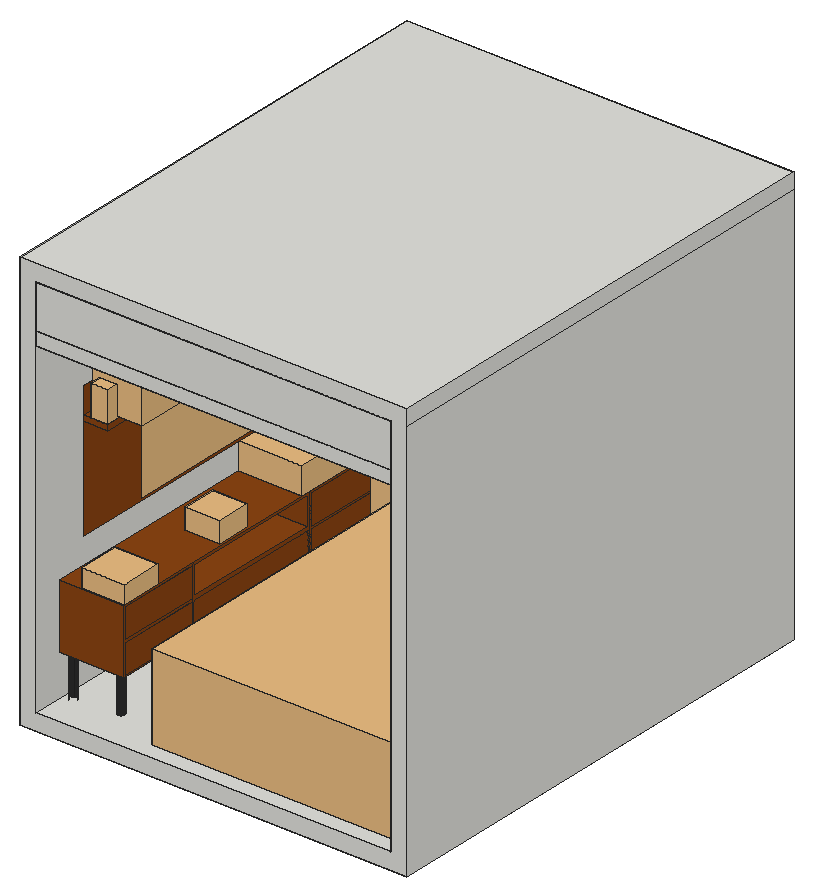
# SketchUp Ruby script. Lengths in inches.
U = 1.inch
M = Sketchup.active_model
def pt(a) = Geom::Point3d.new(a.map { |v| v * U })
def face(e, loops, mat)
  f = e.add_face(loops[0].map { |a| pt(a) })
  loops[1..].each { |l| e.add_face(l.map { |a| pt(a) }).erase! }
  f.material = f.back_material = mat if mat
  f
end
# faces: each face lists its corners as indices into pts; further lists are holes
def faces(e, pts, list, mat = nil) = list.each { |f| face(e, (f[0].is_a?(Array) ? f : [f]).map { |l| l.map { |i| pts[i] } }, mat) }
# xy, xz, yz: faces in a plane at the given z, y or x. An outline is a flat list of corners, or four numbers for a rectangle; further outlines are holes
def ring(l) = l.size == 4 ? [[l[0], l[1]], [l[2], l[1]], [l[2], l[3]], [l[0], l[3]]] : l.each_slice(2).to_a
def flat(e, list, mat, &to3) = list.each { |f| face(e, (f[0].is_a?(Array) ? f : [f]).map { |l| ring(l).map { |u, v| to3.(u, v) } }, mat) }
def xy(e, z, list, mat = nil) = flat(e, list, mat) { |x, y| [x, y, z] }
def xz(e, y, list, mat = nil) = flat(e, list, mat) { |x, z| [x, y, z] }
def yz(e, x, list, mat = nil) = flat(e, list, mat) { |y, z| [x, y, z] }
def lines(e, pts, list) = list.each { |a, b| e.add_line(pt(pts[a]), pt(pts[b])) }
# prism: a flat outline (further loops are holes) pulled along v
def prism(e, loops, v, mat = nil)
  f = face(e, loops, mat); d = Geom::Vector3d.new(v.map { |x| x * U })
  f.pushpull(f.normal.samedirection?(d) ? d.length : -d.length)
end
def box(e, o, s, mat = nil) = prism(e, [[o, [o[0] + s[0], o[1], o[2]], [o[0] + s[0], o[1] + s[1], o[2]], [o[0], o[1] + s[1], o[2]]]], [0, 0, s[2]], mat)
def at(x, y, z, deg = 0) = Geom::Transformation.translation(pt([x, y, z])) * Geom::Transformation.rotation(ORIGIN, Z_AXIS, deg.degrees)
def axes(o, x, y, z) = Geom::Transformation.new([*x, 0, *y, 0, *z, 0, *pt(o).to_a, 1])
def part(name) = M.definitions.add(name)
# library, detail: a bought-in or finely detailed component or shape, given as its bounding box
def library(name, o, s) = part(name).tap { |d| box(d.entities, o, s) }
def detail(e, o, s) = box(e.add_group.entities, o, s)
def put(e, d, t, mat = nil) = e.add_instance(d, t).tap { |i| i.material = mat if mat }
def group(e, t, mat = nil) = e.add_group.tap { |g| g.transformation = t; g.material = mat if mat }.entities
root = M.entities
M.materials.add("0136_Charcoal1").color = [35, 35, 35]
M.materials.add("8").color = [212, 209, 207]
M.materials.add("Glass_Tinted_Gray").color = [0, 0, 0]
M.materials["Glass_Tinted_Gray"].alpha = 0.125
M.materials.add("[0043_SaddleBrown]").color = [139, 69, 19]
M.materials.add("[0135_DarkGray]").color = [81, 81, 81]
M.materials.add("[Color_004]").color = [142, 142, 142]
M.materials.add("[Color_007]").color = [58, 58, 58]
M.materials.add("[Color_C12]").color = [153, 91, 30]
M.materials.add("[Mirror 02]").color = [229, 229, 229]
M.materials.add("[Terrazzo Light Blue]").color = [196, 214, 227]
c1 = library("Group\#15",[-88.79,0.67,-41.3125],[0.99,6.14,4.87])
c2 = library("Group\#18",[-88.79,21.34,-41.3125],[0.99,6.53,4.87])
c3 = library("Group\#19",[-80.46,-65.36,-92.6],[1.38,3.58,3.59])
c4 = library("Group\#9",[-80.34,-149.03,-93.91],[1.18,2.79,3])
c5 = library("Group\#8",[-80.34,-139.83,-93.89],[1.18,2.84,2.98])
c6 = part("Split Brastemp Active 18000")
g1 = group(c6.entities,at(181.47,0,123.23,90))
xy(g1,-123.23,[[-19.69,-181.47,0,181.47]])
xy(g1,-21.89,[[-10.625,-151.65,-8.25,-115.45],[-7.31,-151.65,-4.94,-115.45],[-4,-151.65,-1.63,-115.45],[-10.625,-113.49,-8.25,-77.29],[-7.31,-113.49,-4.94,-77.29],
  [-4,-113.49,-1.63,-77.29],[-10.625,-75.34,-8.25,-39.13],[-7.31,-75.34,-4.94,-39.13],[-4,-75.34,-1.63,-39.13],[-10.625,-37.18,-8.25,-0.98],
  [-7.31,-37.18,-4.94,-0.98],[-4,-37.18,-1.63,-0.98],[-10.625,0.98,-8.25,37.18],[-7.31,0.98,-4.94,37.18],[-4,0.98,-1.63,37.18],
  [-10.625,39.13,-8.25,75.34],[-7.31,39.13,-4.94,75.34],[-4,39.13,-1.63,75.34],[-10.625,77.29,-8.25,113.49],[-7.31,77.29,-4.94,113.49],
  [-4,77.29,-1.63,113.49],[-10.625,115.45,-8.25,151.65],[-7.31,115.45,-4.94,151.65],[-4,115.45,-1.63,151.65]])
xy(g1,0,[[[-19.69,-181.47,0,181.47],[-10.625,39.13,-10.625,113.49,-8.25,113.49,-8.25,77.29,-10.625,77.29,-10.625,75.34,-8.25,75.34,-8.25,39.13],[-4,39.13,-4,75.34,-1.63,75.34,-1.63,77.29,-4,77.29,-4,113.49,-1.63,113.49,-1.63,39.13],[-7.31,115.45,-4.94,151.65],[-4,115.45,-1.63,151.65],[-10.625,115.45,-8.25,151.65],[-10.625,-151.65,-8.25,-115.45],[-4,-151.65,-1.63,-115.45],[-7.31,-151.65,-4.94,-115.45],[-7.31,39.13,-4.94,75.34],[-4,-75.34,-1.63,-39.13],[-7.31,-75.34,-4.94,-39.13],[-10.625,-75.34,-8.25,-39.13],[-7.31,77.29,-4.94,113.49],[-7.31,0.98,-4.94,37.18],[-4,0.98,-1.63,37.18],[-10.625,0.98,-8.25,37.18],[-4,-113.49,-1.63,-77.29],[-10.625,-113.49,-8.25,-77.29],[-10.625,-37.18,-8.25,-0.98],[-7.31,-37.18,-4.94,-0.98],[-4,-37.18,-1.63,-0.98],[-7.31,-113.49,-4.94,-77.29]]])
xz(g1,-181.47,[[-19.69,-123.23,0,0]])
xz(g1,-151.65,[[-10.625,-21.89,-8.25,0],[-7.31,-21.89,-4.94,0],[-4,-21.89,-1.63,0]])
xz(g1,-115.45,[[-10.625,-21.89,-8.25,0],[-7.31,-21.89,-4.94,0],[-4,-21.89,-1.63,0]])
xz(g1,-113.49,[[-10.625,-21.89,-8.25,0],[-7.31,-21.89,-4.94,0],[-4,-21.89,-1.63,0]])
xz(g1,-77.29,[[-10.625,-21.89,-8.25,0],[-7.31,-21.89,-4.94,0],[-4,-21.89,-1.63,0]])
xz(g1,-75.34,[[-10.625,-21.89,-8.25,0],[-7.31,-21.89,-4.94,0],[-4,-21.89,-1.63,0]])
xz(g1,-39.13,[[-10.625,-21.89,-8.25,0],[-7.31,-21.89,-4.94,0],[-4,-21.89,-1.63,0]])
xz(g1,-37.18,[[-10.625,-21.89,-8.25,0],[-7.31,-21.89,-4.94,0],[-4,-21.89,-1.63,0]])
xz(g1,-0.98,[[-10.625,-21.89,-8.25,0],[-7.31,-21.89,-4.94,0],[-4,-21.89,-1.63,0]])
xz(g1,0.98,[[-10.625,-21.89,-8.25,0],[-7.31,-21.89,-4.94,0],[-4,-21.89,-1.63,0]])
xz(g1,37.18,[[-10.625,-21.89,-8.25,0],[-7.31,-21.89,-4.94,0],[-4,-21.89,-1.63,0]])
xz(g1,39.13,[[-10.625,-21.89,-8.25,0],[-7.31,-21.89,-4.94,0],[-4,-21.89,-1.63,0]])
xz(g1,75.34,[[-10.625,-21.89,-8.25,0],[-7.31,-21.89,-4.94,0],[-4,-21.89,-1.63,0]])
xz(g1,77.29,[[-10.625,-21.89,-8.25,0],[-7.31,-21.89,-4.94,0],[-4,-21.89,-1.63,0]])
xz(g1,113.49,[[-10.625,-21.89,-8.25,0],[-7.31,-21.89,-4.94,0],[-4,-21.89,-1.63,0]])
xz(g1,115.45,[[-10.625,-21.89,-8.25,0],[-7.31,-21.89,-4.94,0],[-4,-21.89,-1.63,0]])
xz(g1,151.65,[[-10.625,-21.89,-8.25,0],[-7.31,-21.89,-4.94,0],[-4,-21.89,-1.63,0]])
xz(g1,181.47,[[-19.69,-123.23,0,0]])
yz(g1,-19.69,[[-181.47,-123.23,181.47,0]])
yz(g1,-10.625,[[-151.65,-21.89,-115.45,0],[-113.49,-21.89,-77.29,0],[-75.34,-21.89,-39.13,0],[-37.18,-21.89,-0.98,0],[0.98,-21.89,37.18,0],
  [39.13,-21.89,75.34,0],[77.29,-21.89,113.49,0],[115.45,-21.89,151.65,0]])
yz(g1,-8.25,[[-151.65,-21.89,-115.45,0],[-113.49,-21.89,-77.29,0],[-75.34,-21.89,-39.13,0],[-37.18,-21.89,-0.98,0],[0.98,-21.89,37.18,0],
  [39.13,-21.89,75.34,0],[77.29,-21.89,113.49,0],[115.45,-21.89,151.65,0]])
yz(g1,-7.31,[[-151.65,-21.89,-115.45,0],[-113.49,-21.89,-77.29,0],[-75.34,-21.89,-39.13,0],[-37.18,-21.89,-0.98,0],[0.98,-21.89,37.18,0],
  [39.13,-21.89,75.34,0],[77.29,-21.89,113.49,0],[115.45,-21.89,151.65,0]])
yz(g1,-4.94,[[-151.65,-21.89,-115.45,0],[-113.49,-21.89,-77.29,0],[-75.34,-21.89,-39.13,0],[-37.18,-21.89,-0.98,0],[0.98,-21.89,37.18,0],
  [39.13,-21.89,75.34,0],[77.29,-21.89,113.49,0],[115.45,-21.89,151.65,0]])
yz(g1,-4,[[-151.65,-21.89,-115.45,0],[-113.49,-21.89,-77.29,0],[-75.34,-21.89,-39.13,0],[-37.18,-21.89,-0.98,0],[0.98,-21.89,37.18,0],
  [39.13,-21.89,75.34,0],[77.29,-21.89,113.49,0],[115.45,-21.89,151.65,0]])
yz(g1,-1.63,[[-151.65,-21.89,-115.45,0],[-113.49,-21.89,-77.29,0],[-75.34,-21.89,-39.13,0],[-37.18,-21.89,-0.98,0],[0.98,-21.89,37.18,0],
  [39.13,-21.89,75.34,0],[77.29,-21.89,113.49,0],[115.45,-21.89,151.65,0]])
yz(g1,0,[[-181.47,-123.23,181.47,0]])
g2 = group(c6.entities,at(181.47,0,123.23,90),"[Color_004]")
prism(g2,[[[-87.8,-13.9,-41.3125],[-87.8,-12.33,-41.3125],[-87.8,-13.58,-36.44],[-87.8,-15.625,-36.44],[-87.8,-16.72,-39.72],[-87.8,-17.82,-36.44],[-87.8,-19.78,-36.44],[-87.8,-21.03,-41.3125],[-87.8,-19.46,-41.3125],[-87.8,-18.62,-38.05],[-87.8,-17.58,-41.3125],[-87.8,-15.86,-41.3125],[-87.8,-14.78,-37.9]]],[-1,0,0],"[Color_004]")
put(c6.entities,c1,at(181.47,0,123.23,90))
put(c6.entities,c2,at(181.47,0,123.23,90))
put(c6.entities,c3,at(181.47,-0.89,123.23,90))
g3 = group(c6.entities,at(181.47,0,123.23,90))
detail(g3,[-88.79,14.12,-41.3125],[0.99,6.52,4.87])
g4 = group(c6.entities,at(181.47,0,123.23,90))
detail(g4,[-88.79,-27.6875,-41.3125],[0.99,6.29,4.87])
g5 = group(c6.entities,at(181.47,0,123.23,90))
prism(g5,[[[-87.8,0.21,-37.6],[-87.8,0.21,-36.44],[-87.8,-5.23,-36.44],[-87.8,-5.23,-37.6],[-87.8,-3.45,-37.6],[-87.8,-3.45,-41.3125],[-87.8,-1.66,-41.3125],[-87.8,-1.66,-37.6]]],[-1,0,0],"[Color_004]")
g6 = group(c6.entities,at(181.47,0,123.23,90))
prism(g6,[[[-87.8,181.28,-86.69],[-87.8,181.28,-23.62],[-87.5,181.28,-19.93],[-86.64,181.28,-16.32],[-85.22,181.28,-12.9],[-83.28,181.28,-9.74],[-80.875,181.28,-6.92],[-78.06,181.28,-4.51],[-74.9,181.28,-2.57],[-71.47,181.28,-1.16],[-67.87,181.28,-0.29],[-64.17,181.28,0],[-64.17,181.28,-1.18],[-67.68,181.28,-1.46],[-71.11,181.28,-2.28],[-74.36,181.28,-3.63],[-77.36,181.28,-5.47],[-80.04,181.28,-7.75],[-82.33,181.28,-10.43],[-84.17,181.28,-13.43],[-85.52,181.28,-16.6875],[-86.34,181.28,-20.11],[-86.61,181.28,-23.62],[-86.61,181.28,-86.69]]],[0,-362.55,0])
g7 = group(c6.entities,at(181.47,0,123.23,90))
xy(g7,-119.72,[[-63.45,-153.6,-41.72,153.6]])
xy(g7,-100.82,[[-82.35,-153.6,-79.55,-88.01],[-82.35,-85.65,-79.55,45.54],[-82.35,47.9,-79.55,153.6]])
xy(g7,-95.86,[[-79.55,-153.6,-41.72,-153.6,-41.72,153.6,-79.55,153.6,-79.55,47.9,-82.35,47.9,-82.35,45.54,-79.55,45.54,-79.55,-85.65,-82.35,-85.65,-82.35,-88.01,-79.55,-88.01]])
xz(g7,-153.6,[[-63.45,-119.72,-41.72,-119.72,-41.72,-95.86,-79.55,-95.86,-79.55,-100.82,-82.35,-100.82,-82.32,-101.21,-82.12,-103.78,-81.43,-106.66,-80.29,-109.4,-78.74,-111.93,-76.82,-114.1875,-74.5625,-116.11,-72.03,-117.66,-69.29,-118.8,-66.41,-119.49]])
xz(g7,-88.01,[[-82.35,-100.82,-79.55,-95.86]])
xz(g7,-85.65,[[-82.35,-100.82,-79.55,-95.86]])
xz(g7,45.54,[[-82.35,-100.82,-79.55,-95.86]])
xz(g7,47.9,[[-82.35,-100.82,-79.55,-95.86]])
xz(g7,153.6,[[-63.45,-119.72,-66.41,-119.49,-69.29,-118.8,-72.03,-117.66,-74.5625,-116.11,-76.82,-114.1875,-78.74,-111.93,-80.29,-109.4,-81.43,-106.66,-82.12,-103.78,-82.32,-101.21,-82.35,-100.82,-79.55,-100.82,-79.55,-95.86,-41.72,-95.86,-41.72,-119.72]])
yz(g7,-82.35,[[-88.01,-100.82,-85.65,-95.86],[45.54,-100.82,47.9,-95.86]])
yz(g7,-79.55,[[-153.6,-100.82,-88.01,-95.86],[-85.65,-100.82,45.54,-95.86],[47.9,-100.82,153.6,-95.86]],"[Color_007]")
yz(g7,-41.72,[[-153.6,-119.72,153.6,-95.86]])
p = [[-63.45,153.6,-119.72],[-63.45,-153.6,-119.72],[-66.41,-153.6,-119.49],[-66.41,153.6,-119.49],[-69.29,-153.6,-118.8],[-69.29,153.6,-118.8],
  [-72.03,153.6,-117.66],[-72.03,-153.6,-117.66],[-74.5625,-153.6,-116.11],[-74.5625,153.6,-116.11],[-76.82,-153.6,-114.1875],[-76.82,153.6,-114.1875],
  [-78.74,-153.6,-111.93],[-78.74,153.6,-111.93],[-80.29,-153.6,-109.4],[-80.29,153.6,-109.4],[-81.43,153.6,-106.66],[-81.43,-153.6,-106.66],
  [-82.12,-153.6,-103.78],[-82.12,153.6,-103.78],[-82.32,-153.6,-101.21],[-82.32,-88.01,-101.21],[-82.32,-85.65,-101.21],[-82.32,45.54,-101.21],
  [-82.32,47.9,-101.21],[-82.32,153.6,-101.21],[-82.35,153.6,-100.82],[-82.35,-153.6,-100.82],[-82.35,-88.01,-100.82],[-82.35,-85.65,-100.82],
  [-82.35,45.54,-100.82],[-82.35,47.9,-100.82]]
faces(g7,p,[[0,1,2,3],[4,5,3,2],[6,5,4,7],[6,7,8,9],[10,11,9,8],[11,10,12,13],[14,15,13,12],[16,15,14,17],
  [16,17,18,19],[18,20,21,22,23,24,25,19]])
faces(g7,p,[[26,25,24,23,22,21,20,27,28,29,30,31]],"[Color_C12]")
g8 = group(c6.entities,at(181.47,-0.74,123.23,90))
prism(g8,[[[-80.34,-149.97,-89.91],[-80.34,-149.48,-92.84],[-80.34,-150.15,-92.85],[-80.34,-150.6,-89.91]]],[1.18,0,0],"[Color_004]")
g9 = group(c6.entities,at(181.47,-0.74,123.23,90))
detail(g9,[-80.34,-150.06,-93.9],[1.18,0.73,0.72])
g10 = group(c6.entities,at(181.47,-0.74,123.23,90),"[Color_004]")
prism(g10,[[[-80.34,-145.83,-90.91],[-80.34,-144.76,-92.9],[-80.34,-144.34,-90.91],[-80.34,-143.65,-90.91],[-80.34,-144.28,-93.86],[-80.34,-144.97,-93.86],[-80.34,-146.56,-90.91]]],[1.18,0,0],"[Color_004]")
g11 = group(c6.entities,at(181.47,-0.74,123.23,90))
prism(g11,[[[-80.34,-143.0625,-93.86],[-80.34,-143.55,-90.91],[-80.34,-142.93,-90.91],[-80.34,-142.4,-93.86]]],[1.18,0,0],"[Color_004]")
g12 = group(c6.entities,at(181.47,-0.74,123.23,90))
detail(g12,[-80.34,-143.75,-90.63],[1.18,0.73,0.73])
g13 = group(c6.entities,at(181.47,-0.74,123.23,90))
detail(g13,[-80.34,-142.49,-93.89],[1.18,2.44,3.98])
g14 = group(c6.entities,at(181.47,0,123.23,90))
prism(g14,[[[-87.8,-7.91,-39.48],[-87.8,-7.41,-38.33],[-87.8,-11.11,-38.33],[-87.8,-11.92,-39.48]]],[-1,0,0],"[Color_004]")
put(c6.entities,c4,at(181.47,-0.74,123.23,90))
put(c6.entities,c5,at(181.47,-0.74,123.23,90))
g15 = group(c6.entities,at(181.47,0,123.23,90))
xy(g15,-123.23,[[-64.17,-181.47,-19.69,-153.6],[-64.17,153.6,-19.69,181.47]])
xy(g15,-95.86,[[-79.92,-153.6,-19.69,153.6]])
xy(g15,-93.89,[[-79.92,-33.71,-78.74,33.71]])
xy(g15,-87.73,[[-79.92,-33.71,-78.74,33.71]])
xy(g15,-86.69,[[-87.8,-181.47,-86.61,-153.6],[-86.61,-153.6,-79.92,153.6],[-87.8,153.6,-86.61,181.47]])
xy(g15,0,[[-64.17,-181.47,-19.69,181.47]])
xz(g15,-181.47,[[-64.17,-123.23,-19.69,-123.23,-19.69,0,-64.17,0,-64.17,-1.18,-67.68,-1.46,-71.11,-2.28,-74.36,-3.63,-77.36,-5.47,-80.04,-7.75,-82.33,-10.43,-84.17,-13.43,-85.52,-16.6875,-86.34,-20.11,-86.61,-23.62,-86.61,-86.69,-87.8,-86.69,-87.8,-99.61,-87.5,-103.3,-86.64,-106.91,-85.22,-110.33,-83.28,-113.49,-80.875,-116.31,-78.06,-118.72,-74.9,-120.65,-71.47,-122.07,-67.87,-122.9375]])
xz(g15,-153.6,[[-64.17,-123.23,-67.87,-122.9375,-71.47,-122.07,-74.9,-120.65,-78.06,-118.72,-80.875,-116.31,-83.28,-113.49,-85.22,-110.33,-86.64,-106.91,-87.5,-103.3,-87.8,-99.61,-87.8,-86.69,-79.92,-86.69,-79.92,-95.86,-19.69,-95.86,-19.69,-123.23]])
xz(g15,-33.71,[[-79.92,-93.89,-78.74,-87.73]])
xz(g15,33.71,[[-79.92,-93.89,-78.74,-87.73]])
xz(g15,153.6,[[-64.17,-123.23,-19.69,-123.23,-19.69,-95.86,-79.92,-95.86,-79.92,-86.69,-87.8,-86.69,-87.8,-99.61,-87.5,-103.3,-86.64,-106.91,-85.22,-110.33,-83.28,-113.49,-80.875,-116.31,-78.06,-118.72,-74.9,-120.65,-71.47,-122.07,-67.87,-122.9375]])
xz(g15,181.47,[[-64.17,-123.23,-67.87,-122.9375,-71.47,-122.07,-74.9,-120.65,-78.06,-118.72,-80.875,-116.31,-83.28,-113.49,-85.22,-110.33,-86.64,-106.91,-87.5,-103.3,-87.8,-99.61,-87.8,-86.69,-86.61,-86.69,-86.61,-23.62,-86.34,-20.11,-85.52,-16.6875,-84.17,-13.43,-82.33,-10.43,-80.04,-7.75,-77.36,-5.47,-74.36,-3.63,-71.11,-2.28,-67.68,-1.46,-64.17,-1.18,-64.17,0,-19.69,0,-19.69,-123.23]])
yz(g15,-87.8,[[-181.47,-99.61,-153.6,-86.69],[153.6,-99.61,181.47,-86.69]])
yz(g15,-86.61,[[-181.47,-86.69,181.47,-23.62]])
yz(g15,-79.92,[[[-153.6,-95.86,153.6,-86.69],[-33.71,-93.89,33.71,-87.73]]])
yz(g15,-78.74,[[-33.71,-93.89,33.71,-87.73]],"[Color_007]")
yz(g15,-64.17,[[-181.47,-1.18,181.47,0]])
yz(g15,-19.69,[[-181.47,-123.23,-153.6,-123.23,-153.6,-95.86,153.6,-95.86,153.6,-123.23,181.47,-123.23,181.47,0,-181.47,0]])
p = [[-64.17,-153.6,-123.23],[-64.17,-181.47,-123.23],[-67.87,-181.47,-122.9375],[-67.87,-153.6,-122.9375],[-64.17,181.47,-123.23],[-64.17,153.6,-123.23],
  [-67.87,153.6,-122.9375],[-67.87,181.47,-122.9375],[-71.47,-181.47,-122.07],[-71.47,-153.6,-122.07],[-71.47,153.6,-122.07],[-71.47,181.47,-122.07],
  [-74.9,-153.6,-120.65],[-74.9,-181.47,-120.65],[-74.9,153.6,-120.65],[-74.9,181.47,-120.65],[-78.06,-181.47,-118.72],[-78.06,-153.6,-118.72],
  [-78.06,153.6,-118.72],[-78.06,181.47,-118.72],[-80.875,-181.47,-116.31],[-80.875,-153.6,-116.31],[-80.875,153.6,-116.31],[-80.875,181.47,-116.31],
  [-83.28,-181.47,-113.49],[-83.28,-153.6,-113.49],[-83.28,153.6,-113.49],[-83.28,181.47,-113.49],[-85.22,-181.47,-110.33],[-85.22,-153.6,-110.33],
  [-85.22,153.6,-110.33],[-85.22,181.47,-110.33],[-86.64,-153.6,-106.91],[-86.64,-181.47,-106.91],[-86.64,153.6,-106.91],[-86.64,181.47,-106.91],
  [-87.5,-181.47,-103.3],[-87.5,-153.6,-103.3],[-87.5,153.6,-103.3],[-87.5,181.47,-103.3],[-87.8,-181.47,-99.61],[-87.8,-153.6,-99.61],
  [-87.8,153.6,-99.61],[-87.8,181.47,-99.61],[-86.61,181.47,-23.62],[-86.61,-181.47,-23.62],[-86.34,-181.47,-20.11],[-86.34,181.47,-20.11],
  [-85.52,-181.47,-16.6875],[-85.52,181.47,-16.6875],[-84.17,181.47,-13.43],[-84.17,-181.47,-13.43],[-82.33,-181.47,-10.43],[-82.33,181.47,-10.43],
  [-80.04,-181.47,-7.75],[-80.04,181.47,-7.75],[-77.36,-181.47,-5.47],[-77.36,181.47,-5.47],[-74.36,-181.47,-3.63],[-74.36,181.47,-3.63],
  [-71.11,181.47,-2.28],[-71.11,-181.47,-2.28],[-67.68,-181.47,-1.46],[-67.68,181.47,-1.46],[-64.17,-181.47,-1.18],[-64.17,181.47,-1.18]]
faces(g15,p,[[0,1,2,3],[4,5,6,7],[8,9,3,2],[10,11,7,6],[12,9,8,13],[10,14,15,11],[12,13,16,17],[15,14,18,19],
  [20,21,17,16],[22,23,19,18],[21,20,24,25],[23,22,26,27],[28,29,25,24],[30,31,27,26],[32,29,28,33],[30,34,35,31],
  [32,33,36,37],[35,34,38,39],[40,41,37,36],[42,43,39,38],[44,45,46,47],[48,49,47,46],[50,49,48,51],[50,51,52,53],
  [54,55,53,52],[55,54,56,57],[58,59,57,56],[60,59,58,61],[60,61,62,63],[64,65,63,62]])
g16 = group(c6.entities,at(181.47,0,123.23,90))
prism(g16,[[[-87.8,12.58,-41.3125],[-87.8,14.38,-41.3125],[-87.8,11.73,-36.71],[-87.8,11.67,-36.62],[-87.8,11.58,-36.55],[-87.8,11.49,-36.49],[-87.8,11.38,-36.46],[-87.8,11.27,-36.44],[-87.8,10.0625,-36.44],[-87.8,9.95,-36.46],[-87.8,9.84,-36.49],[-87.8,9.75,-36.55],[-87.8,9.66,-36.62],[-87.8,9.6,-36.71],[-87.8,6.95,-41.3125],[-87.8,8.75,-41.3125],[-87.8,9.34,-40.29],[-87.8,11.99,-40.29]],[[-87.8,11.52,-39.48],[-87.8,9.81,-39.48],[-87.8,10.66,-37.99]]],[-1,0,0],"[Color_004]")
g17 = group(c6.entities,at(181.47,0,123.23,90))
detail(g17,[-88.79,-11.92,-41.3125],[0.99,6.22,4.87])
c7 = part("Untitled (2)")
put(c7.entities,c6,at(0,0,0))
c8 = part("PENTEK_RP Fineline 50S_Sliding_DoorCase_E1")
box(c8.entities,[0,0,0],[1.51,3.66,99.27],"[0135_DarkGray]")
c9 = part("PENTEK_RP Fineline 50S_SlidingDooe_Case_E2")
box(c9.entities,[0,0,0],[96.25,3.66,1.51],"[0135_DarkGray]")
c10 = part("pentek_RP Fineline 50S_SlidingDoor_Case")
put(c10.entities,c8,at(97.76,0,0))
put(c10.entities,c9,at(1.51,0,0))
put(c10.entities,c8,at(0,0,0))
put(c10.entities,c9,at(1.51,0,97.76))
c11 = part("PENTEK_RP Fineline 50S_SlidingDoor_GlazingBead_2")
box(c11.entities,[0,0,0],[0.56,0.59,94.39],"[0135_DarkGray]")
c12 = part("PENTEK_RP Fineline 50S_SlidingDoor_Glass")
box(c12.entities,[0,0,0],[46.58,0.16,94.39],"Glass_Tinted_Gray")
c13 = part("PENTEK_RP Fineline 50S_SlidingDoor_GlazingBead")
box(c13.entities,[0,0,0],[45.47,0.59,0.56],"[0135_DarkGray]")
c14 = part("PENTEK_RP Fineline 50S_SlidingDoor_Leaf_E1")
xy(c14.entities,0,[[0,0,0.93,1.97],[0.93,1.57,1.49,1.97]],"[0135_DarkGray]")
xy(c14.entities,96.25,[[0,0,0.93,0,0.93,1.57,1.49,1.57,1.49,1.97,0,1.97]],"[0135_DarkGray]")
xz(c14.entities,0,[[0,0,0.93,96.25]],"[0135_DarkGray]")
xz(c14.entities,1.57,[[0.93,0,1.49,95.32],[0.93,95.32,1.49,96.25]],"[0135_DarkGray]")
xz(c14.entities,1.97,[[0,0,1.49,96.25]],"[0135_DarkGray]")
yz(c14.entities,0,[[0,0,1.97,96.25]],"[0135_DarkGray]")
yz(c14.entities,0.93,[[0,0,1.57,0.93],[0,0.93,1.57,95.32],[0,95.32,1.57,96.25]],"[0135_DarkGray]")
yz(c14.entities,1.49,[[1.57,0,1.97,95.32],[1.57,95.32,1.97,96.25]],"[0135_DarkGray]")
c15 = part("PENTEK_RP Fineline 50S_SlidingDoor_Leaf_E2")
xy(c15.entities,0,[[0,0,0,1.57,0.56,1.57,0.56,1.97,46.02,1.97,46.02,1.57,46.58,1.57,46.58,0]],"[0135_DarkGray]")
xy(c15.entities,0.93,[[0,0,46.58,1.57]],"[0135_DarkGray]")
xy(c15.entities,1.49,[[0.56,1.57,46.02,1.97]],"[0135_DarkGray]")
xz(c15.entities,0,[[0,0,46.58,0.93]],"[0135_DarkGray]")
xz(c15.entities,1.57,[[0,0,0.56,0.93],[46.02,0,46.58,0.93],[0.56,0.93,46.02,1.49]],"[0135_DarkGray]")
xz(c15.entities,1.97,[[0.56,0,46.02,1.49]],"[0135_DarkGray]")
yz(c15.entities,0,[[0,0,1.57,0.93]],"[0135_DarkGray]")
yz(c15.entities,0.56,[[1.57,0,1.97,0.93],[1.57,0.93,1.97,1.49]],"[0135_DarkGray]")
yz(c15.entities,46.02,[[1.57,0,1.97,0.93],[1.57,0.93,1.97,1.49]],"[0135_DarkGray]")
yz(c15.entities,46.58,[[0,0,1.57,0.93]],"[0135_DarkGray]")
c16 = part("PENTEK_RP Fineline S_SlidingDoor_Leaf1")
put(c16.entities,c11,at(0.93,0,0.93))
put(c16.entities,c11,at(46.96,0,0.93))
put(c16.entities,c12,at(1.49,1.42,0.93))
put(c16.entities,c13,at(1.49,0,0.93))
put(c16.entities,c12,at(1.49,0.59,0.93),"[Terrazzo Light Blue]")
put(c16.entities,c14,at(0,0,0))
put(c16.entities,c14,axes([48.44,0,0],[-1,0,0],[0,1,0],[0,0,1]))
put(c16.entities,c15,axes([0.93,0,96.25],[1,0,0],[0,1,0],[0,0,-1]))
put(c16.entities,c15,at(0.93,0,0))
put(c16.entities,c13,at(1.49,0,94.77))
c17 = part("PENTEK_RP Fineline 50S_SlidingDoor_Leaf2")
put(c17.entities,c12,at(1.49,1.42,0.93))
put(c17.entities,c13,at(1.49,0,94.77))
put(c17.entities,c11,at(46.96,0,0.93))
put(c17.entities,c12,at(1.49,0.59,0.93),"[Mirror 02]")
put(c17.entities,c11,at(0.93,0,0.93))
put(c17.entities,c14,at(0,0,0))
put(c17.entities,c14,axes([48.44,0,0],[-1,0,0],[0,1,0],[0,0,1]))
put(c17.entities,c13,at(1.49,0,0.93))
put(c17.entities,c15,axes([0.93,0,96.25],[1,0,0],[0,1,0],[0,0,-1]))
put(c17.entities,c15,at(0.93,0,0))
c18 = part("PENTEK - Slimmest Steel Sliding Door / Window\#1")
put(c18.entities,c10,at(0,-1.88,-0.09))
put(c18.entities,c16,at(1.51,-2.27,1.42))
put(c18.entities,c17,at(49.32,-0.3,1.42))
c19 = library("8",[-11.64,-17.74,0.06],[182.42,23.72,119.43])
c20 = library("Flat screen television",[0,1.41,1.14],[35.92,0.28,20.21])
c21 = library("Palm",[82.2,-9.29,-2.36],[51.18,55.77,65.42])
c22 = library("Pinch Pot",[-27.95,-27.95,0],[55.9,55.9,47.42])
c23 = part("Potted palm")
put(c23.entities,c21,axes([3796.42,-10488.37,43.97],[0,116.51338,0],[-116.51338,0,0],[0,0,116.51338]))
put(c23.entities,c22,axes([1647.67,1801.1875,0],[0,30.58476,0],[-30.58476,0,0],[0,0,45.1095]))
c24 = library("Untitled (1)",[-27.47,-28.06,0],[55.81,56.64,45.44])
c25 = library("clock",[-2.58,-1.4,-0.01],[5.17,2.61,4.84])
c26 = library("Place setting",[-0.51,0,-0.75],[16.12,15.51,6.82])
c27 = library("Wine glass set",[-12.05,0,0],[27.28,32.06,10.01])
c28 = library("Cup and saucer",[1.11,3.89,0],[6.74,6.75,4.1])
c29 = library("Grupo\#110",[-0.16,-0.24,0],[125.74,135.55,29.78])
c30 = library("Tlon Light 1950 Ceiling 152 010",[-38.39,-38.39,-3.78],[76.78,76.78,3.41])
c31 = library("Group\#39",[-0.5,-0.5,0],[81.67,123.67,1.66])
xy(root,-6,[[0,0,144,180]])
xy(root,-1.51,[[7.66,14.07,7.32,14.12,7,14.25,6.73,14.46,6.52,14.73,6.39,15.04,6.35,15.38,6.39,15.72,6.52,16.04,6.73,16.3125,7,16.52,7.32,16.65,7.66,16.7,8,16.65,8.3125,16.52,8.59,16.3125,8.79,16.04,8.93,15.72,8.97,15.38,8.93,15.04,8.79,14.73,8.59,14.46,8.3125,14.25,8,14.12]])
xy(root,0,[[[6,0,138,0,138,174,6,174,6,165.76,18,165.76,18,125.125,6,125.125],[7.66,122.5,7.32,122.54,7,122.68,6.73,122.88,6.52,123.16,6.39,123.47,6.35,123.8125,6.39,124.15,6.52,124.47,6.73,124.74,7,124.95,7.32,125.08,7.66,125.125,8,125.08,8.3125,124.95,8.59,124.74,8.79,124.47,8.93,124.15,8.97,123.8125,8.93,123.47,8.79,123.16,8.59,122.88,8.3125,122.68,8,122.54],[25.41,14.07,25.07,14.12,24.75,14.25,24.48,14.46,24.27,14.73,24.14,15.04,24.1,15.38,24.14,15.72,24.27,16.04,24.48,16.3125,24.75,16.52,25.07,16.65,25.41,16.7,25.75,16.65,26.0625,16.52,26.34,16.3125,26.54,16.04,26.68,15.72,26.72,15.38,26.68,15.04,26.54,14.73,26.34,14.46,26.0625,14.25,25.75,14.12],[25.41,122.68,25.07,122.72,24.75,122.85,24.48,123.06,24.27,123.33,24.14,123.65,24.1,123.99,24.14,124.33,24.27,124.64,24.48,124.92,24.75,125.125,26.0625,125.125,26.34,124.92,26.54,124.64,26.68,124.33,26.72,123.99,26.68,123.65,26.54,123.33,26.34,123.06,26.0625,122.85,25.75,122.72]]])
xy(root,0.4,[[6,125.52,18,165.36]],"[0043_SaddleBrown]")
xy(root,15.67,[[[6,10.5625,6,125.125,24.75,125.125,24.48,124.92,24.27,124.64,24.14,124.33,24.1,123.99,24.14,123.65,24.27,123.33,24.48,123.06,24.75,122.85,25.07,122.72,25.41,122.68,25.75,122.72,26.0625,122.85,26.34,123.06,26.54,123.33,26.68,123.65,26.72,123.99,26.68,124.33,26.54,124.64,26.34,124.92,26.0625,125.125,30,125.125,30,10.5625],[7.66,122.5,8,122.54,8.3125,122.68,8.59,122.88,8.79,123.16,8.93,123.47,8.97,123.8125,8.93,124.15,8.79,124.47,8.59,124.74,8.3125,124.95,8,125.08,7.66,125.125,7.32,125.08,7,124.95,6.73,124.74,6.52,124.47,6.39,124.15,6.35,123.8125,6.39,123.47,6.52,123.16,6.73,122.88,7,122.68,7.32,122.54],[7.66,14.07,8,14.12,8.3125,14.25,8.59,14.46,8.79,14.73,8.93,15.04,8.97,15.38,8.93,15.72,8.79,16.04,8.59,16.3125,8.3125,16.52,8,16.65,7.66,16.7,7.32,16.65,7,16.52,6.73,16.3125,6.52,16.04,6.39,15.72,6.35,15.38,6.39,15.04,6.52,14.73,6.73,14.46,7,14.25,7.32,14.12],[25.41,14.07,25.75,14.12,26.0625,14.25,26.34,14.46,26.54,14.73,26.68,15.04,26.72,15.38,26.68,15.72,26.54,16.04,26.34,16.3125,26.0625,16.52,25.75,16.65,25.41,16.7,25.07,16.65,24.75,16.52,24.48,16.3125,24.27,16.04,24.14,15.72,24.1,15.38,24.14,15.04,24.27,14.73,24.48,14.46,24.75,14.25,25.07,14.12]]],"[0043_SaddleBrown]")
xy(root,16.27,[[30,97.72,30.6,124.52]],"[0043_SaddleBrown]")
xy(root,16.375,[[30,11.26,30.4,42.05]],"[0043_SaddleBrown]")
xy(root,19.69,[[6,125.52,18,165.36]],"[0043_SaddleBrown]")
xy(root,20.49,[[6,125.52,18,165.36]],"[0043_SaddleBrown]")
xy(root,26.97,[[30,11.26,30.4,42.05]],"[0043_SaddleBrown]")
xy(root,27.07,[[30,97.72,30.6,124.52]],"[0043_SaddleBrown]")
xy(root,28.27,[[30,97.72,30.6,124.52]],"[0043_SaddleBrown]")
xy(root,28.375,[[30,11.26,30.4,42.05],[15.375,43.45,30,96.42]],"[0043_SaddleBrown]")
xy(root,30,[[48,174,108,180]])
xy(root,38.97,[[30,11.26,30.4,42.05],[15.375,43.45,30,96.42]],"[0043_SaddleBrown]")
xy(root,39.07,[[30,97.72,30.6,124.52]],"[0043_SaddleBrown]")
xy(root,39.67,[[6,10.5625,30,125.125]],"[0043_SaddleBrown]")
xy(root,39.79,[[6,125.52,18,165.36]],"[0043_SaddleBrown]")
xy(root,40.59,[[6,125.52,18,165.36]],"[0043_SaddleBrown]")
xy(root,49.79,[[6,21.46,6.5,125.125]],"[0043_SaddleBrown]")
xy(root,59.88,[[6,125.52,18,165.36]],"[0043_SaddleBrown]")
xy(root,60.68,[[6,125.52,18,165.36]],"[0043_SaddleBrown]")
xy(root,79.97,[[6,125.52,18,165.36]],"[0043_SaddleBrown]")
xy(root,80.77,[[6,125.52,18,165.36]],"[0043_SaddleBrown]")
xy(root,88.17,[[6.5,21.46,15.5,125.125]],"[0043_SaddleBrown]")
xy(root,90,[[48,174,108,180]])
xy(root,90.23,[[6.5,21.46,15.5,125.125]],"[0043_SaddleBrown]")
xy(root,99.52,[[6,125.52,18,165.36]],"[0043_SaddleBrown]")
xy(root,99.92,[[6,21.46,6.5,125.125]],"[0043_SaddleBrown]")
xy(root,100.12,[[7.125,125.72,18,130.27],[6,132.04,18,136.02],[6,137.78,18,141.77],[6,143.53,18,147.52],[6,149.28,18,153.27],
  [6,155.03,18,159.01],[6,160.78,18,164.76]],"[0043_SaddleBrown]")
xy(root,117.57,[[6,137.78,18,141.77],[6,143.53,18,147.52],[6,149.28,18,153.27],[6,155.03,18,159.01],[6,160.78,18,164.76]])
xy(root,117.57,[[7.125,125.72,18,130.27],[6,132.04,18,136.02]],"[0043_SaddleBrown]")
xy(root,118.17,[[6,125.125,18,165.76]],"[0043_SaddleBrown]")
xy(root,144,[[6,0,138,174]])
xy(root,150,[[0,0,144,180]])
xz(root,0,[[[0,-6,144,150],[6,0,138,144]],[6,127.63,138,144]])
xz(root,10.5625,[[6,15.67,30,39.67]],"[0043_SaddleBrown]")
xz(root,11.26,[[30,16.375,30.4,26.97],[30,28.375,30.4,38.97]],"[0043_SaddleBrown]")
xz(root,21.46,[[6,49.79,6.5,49.79,6.5,88.17,15.5,88.17,15.5,90.23,6.5,90.23,6.5,99.92,6,99.92]],"[0043_SaddleBrown]")
xz(root,42.05,[[30,16.375,30.4,26.97],[30,28.375,30.4,38.97]],"[0043_SaddleBrown]")
xz(root,43.45,[[15.375,28.375,30,38.97]],"[0043_SaddleBrown]")
xz(root,96.42,[[15.375,28.375,30,38.97]],"[0043_SaddleBrown]")
xz(root,97.72,[[30,16.27,30.6,27.07],[30,28.27,30.6,39.07]],"[0043_SaddleBrown]")
xz(root,124.52,[[30,16.27,30.6,20.09],[30,20.09,30.6,27.07],[30,28.27,30.6,39.07]],"[0043_SaddleBrown]")
xz(root,125.125,[[6,0,7.66,15.67],[24.75,0,26.0625,15.67],[6,15.67,18,39.67],[18,15.67,30,20.09]])
xz(root,125.125,[[7.66,0,18,15.67],[18,20.09,30,39.67],[6,39.67,18,39.67,18,118.17,6,118.17,6,99.92,6.5,99.92,6.5,90.23,15.5,90.23,15.5,88.17,6.5,88.17,6.5,49.79,6,49.79]],"[0043_SaddleBrown]")
xz(root,125.52,[[6,0.4,18,15.67],[6,15.67,18,19.69],[6,39.67,18,39.79]])
xz(root,125.52,[[6,20.49,18,39.67],[6,40.59,18,59.88],[6,60.68,18,79.97],[6,80.77,18,99.52]],"[0043_SaddleBrown]")
xz(root,125.72,[[7.125,100.12,18,117.57]],"[0043_SaddleBrown]")
xz(root,130.27,[[7.125,100.12,18,117.57]],"[0043_SaddleBrown]")
xz(root,132.04,[[6,100.12,18,117.57]],"[0043_SaddleBrown]")
xz(root,136.02,[[6,100.12,18,117.57]],"[0043_SaddleBrown]")
xz(root,137.78,[[6,100.12,18,117.57]],"[0043_SaddleBrown]")
xz(root,141.77,[[6,100.12,18,117.57]],"[0043_SaddleBrown]")
xz(root,143.53,[[6,100.12,18,117.57]],"[0043_SaddleBrown]")
xz(root,147.52,[[6,100.12,18,117.57]],"[0043_SaddleBrown]")
xz(root,149.28,[[6,100.12,18,117.57]],"[0043_SaddleBrown]")
xz(root,153.27,[[6,100.12,18,117.57]],"[0043_SaddleBrown]")
xz(root,155.03,[[6,100.12,18,117.57]],"[0043_SaddleBrown]")
xz(root,159.01,[[6,100.12,18,117.57]],"[0043_SaddleBrown]")
xz(root,160.78,[[6,100.12,18,117.57]],"[0043_SaddleBrown]")
xz(root,164.76,[[6,100.12,18,117.57]],"[0043_SaddleBrown]")
xz(root,165.36,[[6,0.4,18,19.69],[6,20.49,18,39.79],[6,40.59,18,59.88],[6,60.68,18,79.97],[6,80.77,18,99.52]],"[0043_SaddleBrown]")
xz(root,165.76,[[6,0,18,118.17]],"[0043_SaddleBrown]")
xz(root,174,[[[6,0,138,144],[48,30,108,90]]])
xz(root,180,[[[0,-6,144,144],[48,30,108,90]],[0,144,144,150]])
yz(root,0,[[0,-6,180,144],[0,144,180,150]])
yz(root,6,[[0,0,125.125,0,125.125,15.67,10.5625,15.67,10.5625,39.67,125.125,39.67,125.125,49.79,21.46,49.79,21.46,99.92,125.125,99.92,125.125,118.17,165.76,118.17,165.76,0,174,0,174,144,0,144]])
yz(root,6,[[125.52,0.4,165.36,19.69],[125.52,20.49,165.36,39.79],[125.52,40.59,165.36,59.88],[125.52,60.68,165.36,79.97],[125.52,80.77,165.36,99.52],
  [132.04,100.12,136.02,117.57],[137.78,100.12,141.77,117.57],[143.53,100.12,147.52,117.57],[149.28,100.12,153.27,117.57],[155.03,100.12,159.01,117.57],
  [160.78,100.12,164.76,117.57]],"[0043_SaddleBrown]")
yz(root,6.5,[[21.46,49.79,125.125,88.17],[21.46,90.23,125.125,99.92]],"[0043_SaddleBrown]")
yz(root,7.125,[[125.72,100.12,130.27,117.57]],"[0043_SaddleBrown]")
yz(root,15.375,[[43.45,28.375,96.42,38.97]],"[0043_SaddleBrown]")
yz(root,15.5,[[21.46,88.17,125.125,90.23]],"[0043_SaddleBrown]")
yz(root,18,[[[125.125,0,165.76,0,165.76,99.52,165.36,99.52,165.36,80.77,125.52,80.77,125.52,99.52,125.125,99.52],[125.52,20.49,165.36,39.79],[125.52,40.59,165.36,59.88],[125.52,0.4,165.36,19.69],[125.52,60.68,165.36,79.97]],[[125.125,99.52,165.76,118.17],[125.72,100.12,130.27,117.57],[132.04,100.12,136.02,117.57],[155.03,100.12,159.01,117.57],[137.78,100.12,141.77,117.57],[143.53,100.12,147.52,117.57],[149.28,100.12,153.27,117.57],[160.78,100.12,164.76,117.57]]],"[0043_SaddleBrown]")
yz(root,30,[[[10.5625,15.67,42.75,39.67],[11.26,16.375,42.05,26.97],[11.26,28.375,42.05,38.97]],[[42.75,15.67,97.125,39.67],[43.45,16.375,96.42,26.97],[43.45,28.375,96.42,38.97]],[[97.125,15.67,125.125,39.67],[97.72,16.27,124.52,27.07],[97.72,28.27,124.52,39.07]],[43.45,16.375,96.42,26.97]],"[0043_SaddleBrown]")
yz(root,30.4,[[11.26,16.375,42.05,26.97],[11.26,28.375,42.05,38.97]],"[0043_SaddleBrown]")
yz(root,30.6,[[97.72,16.27,124.52,27.07],[97.72,28.27,124.52,39.07]],"[0043_SaddleBrown]")
yz(root,48,[[174,30,180,90]])
yz(root,108,[[174,30,180,90]])
yz(root,138,[[0,0,174,144]])
yz(root,144,[[0,-6,180,144],[0,144,180,150]])
p = [[7.32,14.12,15.67],[7,14.25,15.67],[7,14.25,-1.51],[7.32,14.12,-1.51],[7.66,14.07,15.67],[7.66,14.07,-1.51],
  [8,14.12,15.67],[8,14.12,-1.51],[8.3125,14.25,15.67],[8.3125,14.25,-1.51],[6.73,14.46,15.67],[6.73,14.46,-1.51],
  [8.59,14.46,15.67],[8.59,14.46,-1.51],[6.52,14.73,15.67],[6.52,14.73,-1.51],[8.79,14.73,15.67],[8.79,14.73,-1.51],
  [6.39,15.04,15.67],[6.39,15.04,-1.51],[8.93,15.04,15.67],[8.93,15.04,-1.51],[6.35,15.38,15.67],[6.35,15.38,-1.51],
  [8.97,15.38,15.67],[8.97,15.38,-1.51],[6.39,15.72,15.67],[6.39,15.72,-1.51],[8.93,15.72,15.67],[8.93,15.72,-1.51],
  [6.52,16.04,15.67],[6.52,16.04,-1.51],[8.79,16.04,15.67],[8.79,16.04,-1.51],[6.73,16.3125,15.67],[6.73,16.3125,-1.51],
  [8.59,16.3125,15.67],[8.59,16.3125,-1.51],[7,16.52,15.67],[7,16.52,-1.51],[8.3125,16.52,15.67],[8.3125,16.52,-1.51],
  [7.32,16.65,15.67],[7.32,16.65,-1.51],[8,16.65,15.67],[8,16.65,-1.51],[7.66,16.7,15.67],[7.66,16.7,-1.51],
  [25.07,14.12,15.67],[24.75,14.25,15.67],[24.75,14.25,0],[25.07,14.12,0],[25.41,14.07,15.67],[25.41,14.07,0],
  [25.75,14.12,15.67],[25.75,14.12,0],[26.0625,14.25,15.67],[26.0625,14.25,0],[24.48,14.46,15.67],[24.48,14.46,0],
  [26.34,14.46,15.67],[26.34,14.46,0],[24.27,14.73,15.67],[24.27,14.73,0],[26.54,14.73,15.67],[26.54,14.73,0],
  [24.14,15.04,15.67],[24.14,15.04,0],[26.68,15.04,15.67],[26.68,15.04,0],[24.1,15.38,15.67],[24.1,15.38,0],
  [26.72,15.38,15.67],[26.72,15.38,0],[24.14,15.72,15.67],[24.14,15.72,0],[26.68,15.72,15.67],[26.68,15.72,0],
  [24.27,16.04,15.67],[24.27,16.04,0],[26.54,16.04,15.67],[26.54,16.04,0],[24.48,16.3125,15.67],[24.48,16.3125,0],
  [26.34,16.3125,15.67],[26.34,16.3125,0],[24.75,16.52,15.67],[24.75,16.52,0],[26.0625,16.52,15.67],[26.0625,16.52,0],
  [25.07,16.65,15.67],[25.07,16.65,0],[25.75,16.65,15.67],[25.75,16.65,0],[25.41,16.7,15.67],[25.41,16.7,0],
  [7.32,122.54,15.67],[7,122.68,15.67],[7,122.68,0],[7.32,122.54,0],[7.66,122.5,15.67],[7.66,122.5,0],
  [8,122.54,15.67],[8,122.54,0],[8.3125,122.68,15.67],[8.3125,122.68,0],[6.73,122.88,15.67],[6.73,122.88,0],
  [8.59,122.88,15.67],[8.59,122.88,0],[25.07,122.72,15.67],[24.75,122.85,15.67],[24.75,122.85,0],[25.07,122.72,0],
  [25.41,122.68,15.67],[25.41,122.68,0],[25.75,122.72,15.67],[25.75,122.72,0],[26.0625,122.85,15.67],[26.0625,122.85,0],
  [6.52,123.16,15.67],[6.52,123.16,0],[8.79,123.16,15.67],[8.79,123.16,0],[24.48,123.06,15.67],[24.48,123.06,0],
  [26.34,123.06,15.67],[26.34,123.06,0],[24.27,123.33,15.67],[24.27,123.33,0],[26.54,123.33,15.67],[26.54,123.33,0],
  [6.39,123.47,15.67],[6.39,123.47,0],[8.93,123.47,15.67],[8.93,123.47,0],[24.14,123.65,15.67],[24.14,123.65,0],
  [26.68,123.65,15.67],[26.68,123.65,0],[6.35,123.8125,15.67],[6.35,123.8125,0],[8.97,123.8125,15.67],[8.97,123.8125,0],
  [24.1,123.99,15.67],[24.1,123.99,0],[26.72,123.99,15.67],[26.72,123.99,0],[6.39,124.15,15.67],[6.39,124.15,0],
  [8.93,124.15,15.67],[8.93,124.15,0],[24.14,124.33,15.67],[24.14,124.33,0],[26.68,124.33,15.67],[26.68,124.33,0],
  [6.52,124.47,15.67],[6.52,124.47,0],[8.79,124.47,15.67],[8.79,124.47,0],[24.27,124.64,15.67],[24.27,124.64,0],
  [26.54,124.64,15.67],[26.54,124.64,0],[6.73,124.74,15.67],[6.73,124.74,0],[8.59,124.74,15.67],[8.59,124.74,0],
  [24.48,124.92,15.67],[24.48,124.92,0],[26.34,124.92,15.67],[26.34,124.92,0],[7,124.95,15.67],[7,124.95,0],
  [8.3125,124.95,15.67],[8.3125,124.95,0],[7.32,125.08,15.67],[7.32,125.08,0],[8,125.08,15.67],[8,125.08,0],
  [24.75,125.125,15.67],[24.75,125.125,0],[26.0625,125.125,15.67],[26.0625,125.125,0],[7.66,125.125,15.67],[7.66,125.125,0]]
faces(root,p,[[0,1,2,3],[4,0,3,5],[6,4,5,7],[8,6,7,9],[1,10,11,2],[12,8,9,13],[10,14,15,11],[16,12,13,17],
  [14,18,19,15],[20,16,17,21],[18,22,23,19],[24,20,21,25],[22,26,27,23],[28,24,25,29],[26,30,31,27],[32,28,29,33],
  [30,34,35,31],[36,32,33,37],[34,38,39,35],[40,36,37,41],[38,42,43,39],[44,40,41,45],[42,46,47,43],[46,44,45,47],
  [48,49,50,51],[52,48,51,53],[54,52,53,55],[56,54,55,57],[49,58,59,50],[60,56,57,61],[58,62,63,59],[64,60,61,65],
  [62,66,67,63],[68,64,65,69],[66,70,71,67],[72,68,69,73],[70,74,75,71],[76,72,73,77],[74,78,79,75],[80,76,77,81],
  [78,82,83,79],[84,80,81,85],[82,86,87,83],[88,84,85,89],[86,90,91,87],[92,88,89,93],[90,94,95,91],[94,92,93,95],
  [96,97,98,99],[100,96,99,101],[102,100,101,103],[104,102,103,105],[97,106,107,98],[108,104,105,109],[110,111,112,113],[114,110,113,115],
  [116,114,115,117],[118,116,117,119],[106,120,121,107],[122,108,109,123],[111,124,125,112],[126,118,119,127],[124,128,129,125],[130,126,127,131],
  [120,132,133,121],[134,122,123,135],[128,136,137,129],[138,130,131,139],[132,140,141,133],[142,134,135,143],[136,144,145,137],[146,138,139,147],
  [140,148,149,141],[150,142,143,151],[144,152,153,145],[154,146,147,155],[148,156,157,149],[158,150,151,159],[152,160,161,153],[162,154,155,163],
  [156,164,165,157],[166,158,159,167],[160,168,169,161],[170,162,163,171],[164,172,173,165],[174,166,167,175],[172,176,177,173],[178,174,175,179],
  [168,180,181,169],[182,170,171,183],[176,184,185,177],[184,178,179,185]],"0136_Charcoal1")
put(root,c7,axes([138,122.66,82.19],[0,-0.19,0],[0.19,0,0],[0,0,0.19]))
put(root,c18,axes([48.95,178.9375,31.01],[0.5948,0,0],[0,0.5948,0],[0,0,0.5948]))
put(root,c19,axes([52.04,175.03,21.83],[0.34669,0,0],[0,1.02131,0],[0,0,0.6051]))
put(root,c20,axes([9.02,48.3,48.99],[0,1.72,0],[-1.72,0,0],[0,0,1.72]))
put(root,c23,axes([21.96,142.07,2.28],[0.00986,0,0],[0,0.00986,0],[0,0,0.00986]))
put(root,c24,axes([12.53,37.8125,91.25],[0.4312,0,0],[0,0.4312,0],[0,0,0.4312]))
put(root,c24,axes([10.47,64.0625,91.25],[0.4312,0,0],[0,0.4312,0],[0,0,0.4312]))
put(root,c24,axes([11.34,101.41,91.32],[0.46,0,0],[0,0.46,0],[0,0,0.46]))
put(root,c25,axes([12.14,27.76,90.26],[0,2.4,0],[-2.4,0,0],[0,0,2.4]))
put(root,c26,at(14.39,11.14,40.42))
put(root,c27,at(14.64,93.92,39.67))
put(root,c28,axes([14.05,49.34,39.67],[1.89,0,0],[0,1.89,0],[0,0,1.89]))
put(root,c26,at(2.39,137.29,40.53))
put(root,c29,axes([43.82,6.74,-0.23],[0.75,0,0],[0,1.2644,0],[0,0,1.07745]))
g18 = group(root,at(6,0,122.26))
xy(g18,0.375,[[[0,0,132,174],[26.07,26.07,105.93,147.93]]])
xy(g18,2.03,[[25.67,25.67,106.33,26.07],[25.67,26.07,26.07,148.33],[105.93,26.07,106.33,148.33],[26.07,147.93,105.93,148.33]])
xy(g18,3.6875,[[25.67,25.67,106.33,148.33]])
xy(g18,5.375,[[0,0,132,174]])
xz(g18,0,[[0,0.375,132,5.375]])
xz(g18,26.07,[[26.07,0.375,105.93,2.03]])
xz(g18,147.93,[[26.07,0.375,105.93,2.03]])
xz(g18,174,[[0,0.375,132,5.375]])
yz(g18,0,[[0,0.375,174,5.375]])
yz(g18,26.07,[[26.07,0.375,147.93,2.03]])
yz(g18,105.93,[[26.07,0.375,147.93,2.03]])
yz(g18,132,[[0,0.375,174,5.375]])
put(g18,c30,axes([15.48,95.03,0.79],[0.11,0,0],[0,0.11,0],[0,0,0.11]))
put(g18,c30,axes([15.48,154.53,0.79],[0.11,0,0],[0,0.11,0],[0,0,0.11]))
put(g18,c30,axes([66.92,11.13,0.79],[0.11,0,0],[0,0.11,0],[0,0,0.11]))
put(g18,c30,axes([119.73,154.53,0.79],[0.11,0,0],[0,0.11,0],[0,0,0.11]))
put(g18,c30,axes([65.17,154.53,0.79],[0.11,0,0],[0,0.11,0],[0,0,0.11]))
put(g18,c30,axes([119.73,16.41,0.79],[0.11,0,0],[0,0.11,0],[0,0,0.11]))
put(g18,c30,axes([119.73,78.97,0.79],[0.11,0,0],[0,0.11,0],[0,0,0.11]))
put(g18,c30,axes([14.75,12.05,0.42],[0.11,0,0],[0,0.11,0],[0,0,0.11]))
put(g18,c31,at(25.67,25.67,2.03))
